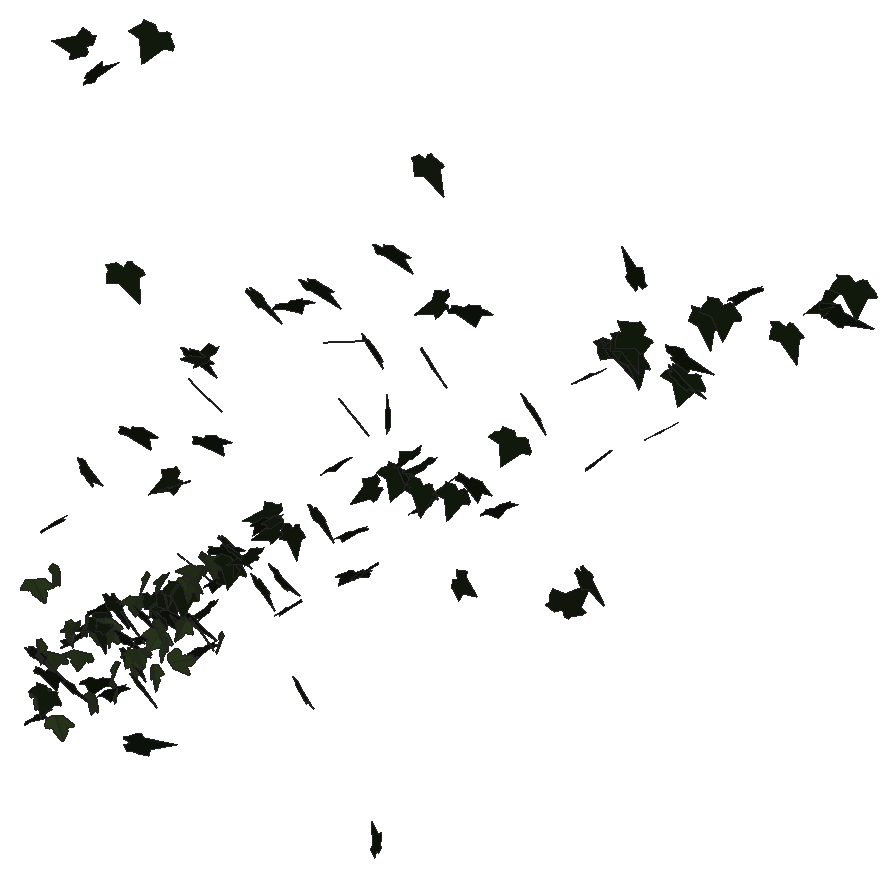
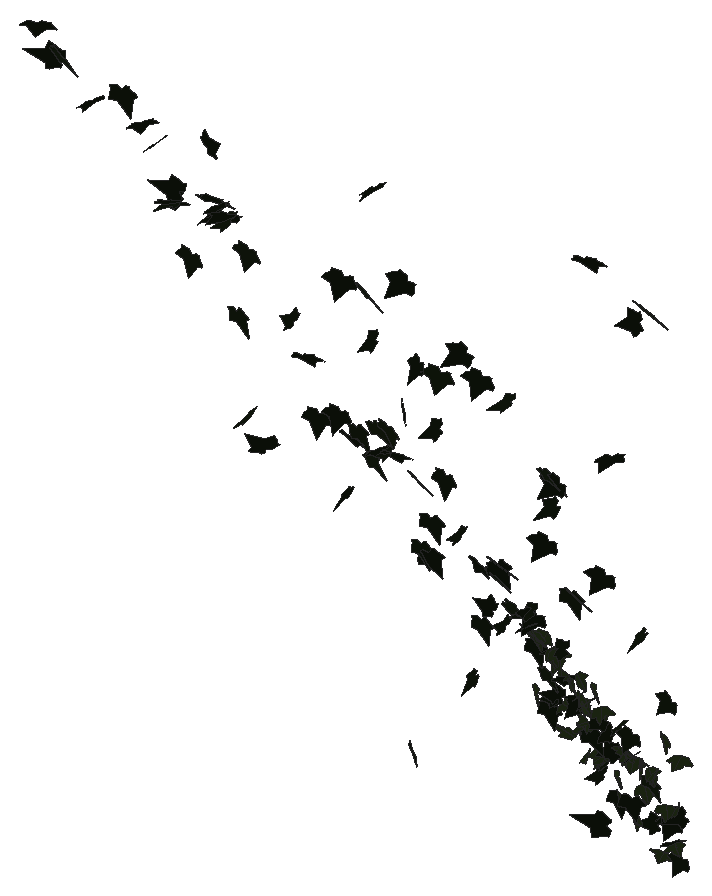
# SketchUp Ruby script. Lengths in inches.
U = 1.inch
M = Sketchup.active_model
def pt(a) = Geom::Point3d.new(a.map { |v| v * U })
def face(e, loops, mat)
  f = e.add_face(loops[0].map { |a| pt(a) })
  loops[1..].each { |l| e.add_face(l.map { |a| pt(a) }).erase! }
  f.material = f.back_material = mat if mat
  f
end
# faces: each face lists its corners as indices into pts; further lists are holes
def faces(e, pts, list, mat = nil) = list.each { |f| face(e, (f[0].is_a?(Array) ? f : [f]).map { |l| l.map { |i| pts[i] } }, mat) }
# xy, xz, yz: faces in a plane at the given z, y or x. An outline is a flat list of corners, or four numbers for a rectangle; further outlines are holes
def ring(l) = l.size == 4 ? [[l[0], l[1]], [l[2], l[1]], [l[2], l[3]], [l[0], l[3]]] : l.each_slice(2).to_a
def flat(e, list, mat, &to3) = list.each { |f| face(e, (f[0].is_a?(Array) ? f : [f]).map { |l| ring(l).map { |u, v| to3.(u, v) } }, mat) }
def xy(e, z, list, mat = nil) = flat(e, list, mat) { |x, y| [x, y, z] }
def xz(e, y, list, mat = nil) = flat(e, list, mat) { |x, z| [x, y, z] }
def yz(e, x, list, mat = nil) = flat(e, list, mat) { |y, z| [x, y, z] }
def lines(e, pts, list) = list.each { |a, b| e.add_line(pt(pts[a]), pt(pts[b])) }
# prism: a flat outline (further loops are holes) pulled along v
def prism(e, loops, v, mat = nil)
  f = face(e, loops, mat); d = Geom::Vector3d.new(v.map { |x| x * U })
  f.pushpull(f.normal.samedirection?(d) ? d.length : -d.length)
end
def box(e, o, s, mat = nil) = prism(e, [[o, [o[0] + s[0], o[1], o[2]], [o[0] + s[0], o[1] + s[1], o[2]], [o[0], o[1] + s[1], o[2]]]], [0, 0, s[2]], mat)
def at(x, y, z, deg = 0) = Geom::Transformation.translation(pt([x, y, z])) * Geom::Transformation.rotation(ORIGIN, Z_AXIS, deg.degrees)
def axes(o, x, y, z) = Geom::Transformation.new([*x, 0, *y, 0, *z, 0, *pt(o).to_a, 1])
def part(name) = M.definitions.add(name)
# library, detail: a bought-in or finely detailed component or shape, given as its bounding box
def library(name, o, s) = part(name).tap { |d| box(d.entities, o, s) }
def detail(e, o, s) = box(e.add_group.entities, o, s)
def put(e, d, t, mat = nil) = e.add_instance(d, t).tap { |i| i.material = mat if mat }
def group(e, t, mat = nil) = e.add_group.tap { |g| g.transformation = t; g.material = mat if mat }.entities
root = M.entities
M.materials.add("1026 AP 7946 SUNNY SIDE UP").color = [254, 231, 186]
M.materials.add("efeu1").color = [18, 25, 13]
M.materials.add("efeu2").color = [43, 57, 29]
c1 = part("ivyleaf_10")
p = [[0,0.5,-0.03],[-0.0625,2.02,-0.43],[-0.19,2.01,-0.46],[-0.54,1.05,-0.29],[-0.52,0.625,-0.18],[-0.83,0.76,-0.28],
  [-1.16,0.64,-0.33],[-1.15,0.33,-0.24],[-0.77,-0.39,0.02],[-0.3,-0.51,0.16],[0.04,-0.48,0.23],[-0.02,2.01,-0.4375],
  [-0.06,2.01,-0.43],[0.04,-0.49,0.23],[0.67,-0.49,0.14],[1.38,0.36,-0.2],[1.375,0.51,-0.24],[0.81,0.65,-0.19],
  [0.62,0.59,-0.15],[0.6,1.09,-0.28],[0.5,1.23,-0.31]]
faces(c1.entities,p,[[0,1,2,3,4,5,6,7,8,9,10],[11,12,0,13,14,15,16,17,18,19,20]],"efeu2")
c2 = part("ivyleaf_9")
p = [[1.54,2.16,1.25],[1.36,2.04,1.19],[-0.21,0.99,0.68],[-0.71,1.11,0.82],[-0.85,0.86,0.67],[-0.8,0.17,0.21],
  [-0.9,-0.01,0.1],[-0.67,-0.16,-0.02],[-0.08,-0.08,-0.05],[-0.03,-0.6,-0.4],[0.65,-0.88,-0.66],[0.83,-0.6,-0.49],
  [1.29,-0.42,-0.43],[1.8125,-0.07,-0.26],[1.21,0.44,0.15]]
faces(c2.entities,p,[[0,1,2,3,4,5,6,7,8,9,10,11,12,13,14]],"efeu1")
put(root,c1,axes([152.7,212.68,300.75],[-0.46729,-0.23939,-0.10574],[0.24139,-0.0375,-0.37295],[0.32982,-0.31172,0.12315]),"1026 AP 7946 SUNNY SIDE UP")
put(root,c2,axes([152.8,212.41,294.52],[0.19714,0.31739,0.16916],[0.09359,0.15111,-0.35068],[-0.55274,0.13879,0.00096]),"1026 AP 7946 SUNNY SIDE UP")
put(root,c1,axes([152.82,212.89,295.55],[0.30918,0.29061,-0.12024],[-0.13325,-0.08531,-0.36131],[-0.47507,0.21306,0.02309]),"1026 AP 7946 SUNNY SIDE UP")
put(root,c2,axes([152.45,212.77,297.4],[0.57206,-0.07756,0.06933],[0.08895,-0.05728,-0.38092],[0.13529,0.3656,-0.04269]),"1026 AP 7946 SUNNY SIDE UP")
put(root,c1,axes([152.77,212.8,297.81],[-0.08655,0.35409,-0.1255],[0.01107,-0.12416,-0.3697],[-0.58974,-0.05429,0.01148]),"1026 AP 7946 SUNNY SIDE UP")
put(root,c2,axes([153.16,212.88,295.63],[-0.25478,-0.32974,0.04474],[0.01184,-0.05401,-0.37752],[0.52322,-0.15934,0.03033]),"1026 AP 7946 SUNNY SIDE UP")
put(root,c2,axes([153.25,212.65,296.75],[0.51975,0.11539,-0.12956],[-0.17017,-0.07208,-0.35973],[-0.2085,0.34647,-0.02935]),"1026 AP 7946 SUNNY SIDE UP")
put(root,c1,axes([153.52,212.82,297.53],[-0.51807,-0.17242,0.03289],[-0.02153,-0.04451,-0.38185],[0.27517,-0.32811,0.03204]),"1026 AP 7946 SUNNY SIDE UP")
put(root,c2,axes([153.55,212.47,303.86],[0.22967,0.2776,0.26829],[0.13322,0.24652,-0.32016],[-0.58177,0.16604,0.0326]),"1026 AP 7946 SUNNY SIDE UP")
put(root,c1,axes([153.77,212.6875,301.67],[0.42896,-0.28302,-0.06521],[0.00837,0.08964,-0.39882],[0.4554,0.26494,0.06876]),"1026 AP 7946 SUNNY SIDE UP")
put(root,c1,axes([153.8,212.67,294.61],[0.5271,0.1067,0.13398],[0.20634,0.01343,-0.36139],[-0.16433,0.35909,-0.02401]),"1026 AP 7946 SUNNY SIDE UP")
put(root,c2,axes([154.73,212.72,298.75],[-0.13124,0.37251,0.05344],[-0.11374,0.03409,-0.38775],[-0.57989,-0.09099,0.06396]),"1026 AP 7946 SUNNY SIDE UP")
put(root,c1,axes([154.41,212.6875,299.27],[-0.05091,0.38742,-0.02757],[-0.00042,-0.02908,-0.40067],[-0.61088,-0.03226,0.00257]),"1026 AP 7946 SUNNY SIDE UP")
put(root,c1,axes([154.61,212.78,299.37],[-0.08768,-0.38044,0.04128],[-0.0053,-0.04219,-0.39635],[0.60185,-0.0558,0.00253]),"1026 AP 7946 SUNNY SIDE UP")
put(root,c2,axes([154.125,212.89,296.4],[0.43646,-0.17986,0.1778],[0.2205,-0.10272,-0.34122],[0.32539,0.31086,-0.00725]),"1026 AP 7946 SUNNY SIDE UP")
put(root,c2,axes([155.28,212.65,327.21],[-0.43062,0.331,0.19807],[-0.30187,0.08317,-0.43297],[-0.51901,-0.323,0.08749]),"1026 AP 7946 SUNNY SIDE UP")
put(root,c1,axes([155.05,212.71,298.16],[-0.45669,-0.23847,0.06481],[-0.04426,-0.06659,-0.38603],[0.38582,-0.28992,0.03243]),"1026 AP 7946 SUNNY SIDE UP")
put(root,c1,axes([155.23,212.79,299.65],[0.16583,-0.3476,-0.13742],[0.0593,0.14591,-0.36556],[0.5813,0.08427,0.07649]),"1026 AP 7946 SUNNY SIDE UP")
put(root,c2,axes([155.34,212.46,307.31],[0.47061,-0.11988,-0.26885],[-0.29648,0.20104,-0.31756],[0.33932,0.34192,0.0954]),"1026 AP 7946 SUNNY SIDE UP")
put(root,c1,axes([155.68,212.71,296.28],[0.45432,-0.24443,-0.03533],[0.03609,0.07711,-0.38202],[0.38612,0.28039,0.07728]),"1026 AP 7946 SUNNY SIDE UP")
put(root,c2,axes([155.87,212.76,297.23],[0.21645,0.30392,-0.18263],[-0.09119,-0.17003,-0.34435],[-0.54706,0.14859,-0.01486]),"1026 AP 7946 SUNNY SIDE UP")
put(root,c1,axes([155.89,212.75,299.67],[-0.56757,-0.12501,-0.00205],[0.01887,-0.03075,-0.39224],[0.19567,-0.35965,0.03187]),"1026 AP 7946 SUNNY SIDE UP")
put(root,c2,axes([156.25,212.89,300.09],[-0.57953,0.1147,0.01403],[-0.0702,-0.10162,-0.38169],[-0.16737,-0.35452,0.11149]),"1026 AP 7946 SUNNY SIDE UP")
put(root,c2,axes([155.74,212.46,326.01],[0.20754,0.14293,0.43993],[0.40404,0.34051,-0.19762],[-0.58002,0.28834,0.01976]),"1026 AP 7946 SUNNY SIDE UP")
put(root,c2,axes([155.84,212.85,299.84],[0.07382,-0.38326,0.00387],[-0.01214,-0.00692,-0.39773],[0.60259,0.04681,-0.00849]),"1026 AP 7946 SUNNY SIDE UP")
put(root,c2,axes([156.17,212.43,300.89],[0.24256,0.34415,0.13491],[0.07431,0.12017,-0.38778],[-0.57311,0.16123,0.00682]),"1026 AP 7946 SUNNY SIDE UP")
put(root,c1,axes([156.32,212.91,299.84],[-0.38888,0.27151,-0.11323],[-0.00772,-0.14955,-0.36498],[-0.46143,-0.22632,0.10153]),"1026 AP 7946 SUNNY SIDE UP")
put(root,c1,axes([156.26,212.87,300.02],[-0.51042,-0.01549,-0.21285],[0.30783,-0.14824,-0.30641],[-0.10626,-0.35504,0.13477]),"1026 AP 7946 SUNNY SIDE UP")
put(root,c2,axes([156.75,212.6875,297.1],[0.13138,0.36736,-0.06784],[-0.00435,-0.06901,-0.38831],[-0.58742,0.08267,-0.0123]),"1026 AP 7946 SUNNY SIDE UP")
put(root,c1,axes([156.85,212.71,297.16],[0.31676,-0.29345,-0.14725],[-0.00811,0.16321,-0.35589],[0.51203,0.18412,0.08545]),"1026 AP 7946 SUNNY SIDE UP")
put(root,c1,axes([156.875,212.77,298.21],[0.29073,-0.29999,0.15478],[0.10385,-0.13763,-0.36352],[0.51846,0.19579,-0.01398]),"1026 AP 7946 SUNNY SIDE UP")
put(root,c2,axes([156.65,212.76,301.36],[0.26644,-0.35465,-0.03665],[0.00569,0.03888,-0.40417],[0.56012,0.16831,0.02154]),"1026 AP 7946 SUNNY SIDE UP")
put(root,c2,axes([156.99,212.8,299.73],[0.53572,-0.10857,0.15097],[0.21563,-0.05418,-0.36857],[0.19023,0.36715,-0.00737]),"1026 AP 7946 SUNNY SIDE UP")
put(root,c2,axes([157.38,212.64,317.38],[-0.05948,-0.3931,-0.27522],[0.04293,0.26351,-0.4053],[0.74414,-0.04663,0.00138]),"1026 AP 7946 SUNNY SIDE UP")
put(root,c2,axes([157.42,212.68,300.78],[0.52894,-0.17181,-0.08172],[-0.13092,0.00871,-0.38789],[0.26649,0.34528,-0.02836]),"1026 AP 7946 SUNNY SIDE UP")
put(root,c2,axes([157.41,212.89,299.02],[0.2769,-0.33735,-0.04186],[-0.00069,0.04339,-0.39126],[0.53393,0.175,0.0212]),"1026 AP 7946 SUNNY SIDE UP")
put(root,c1,axes([157.8,212.68,298.99],[0.1388,0.37292,0.00465],[0.00614,0.00153,-0.39477],[-0.58635,0.08829,-0.00304]),"1026 AP 7946 SUNNY SIDE UP")
put(root,c1,axes([158,212.72,301.83],[-0.36108,-0.32324,0.00717],[0.0594,-0.03753,-0.4051],[0.50497,-0.22672,0.05278]),"1026 AP 7946 SUNNY SIDE UP")
put(root,c1,axes([157.95,212.79,299.27],[-0.4155,-0.2615,-0.10896],[0.16797,0.03919,-0.37988],[0.40957,-0.28136,0.04525]),"1026 AP 7946 SUNNY SIDE UP")
put(root,c2,axes([157.94,212.5,309.96],[0.59891,0.18821,-0.04457],[-0.03454,-0.05519,-0.4361],[-0.30207,0.37947,-0.0385]),"1026 AP 7946 SUNNY SIDE UP")
put(root,c2,axes([157.87,212.73,301.35],[0.58966,-0.11928,0.0099],[0.00204,-0.02978,-0.40455],[0.18824,0.37396,-0.02663]),"1026 AP 7946 SUNNY SIDE UP")
put(root,c2,axes([157.95,212.72,298],[0.4141,-0.27586,0.05587],[0.04931,-0.04719,-0.39305],[0.43979,0.26504,-0.00854]),"1026 AP 7946 SUNNY SIDE UP")
put(root,c2,axes([157.81,212.67,294.98],[0.3582,0.23468,-0.33496],[0.26032,0.2872,0.33337],[0.57614,-0.27568,0.05762]),"1026 AP 7946 SUNNY SIDE UP")
put(root,c2,axes([158.58,212.78,300.3],[0.00189,0.34594,-0.17418],[-0.09662,-0.16868,-0.35292],[-0.59907,0.0283,0.05637]),"1026 AP 7946 SUNNY SIDE UP")
put(root,c1,axes([158.51,212.73,302.99],[0.27732,-0.35602,0.04732],[0.01368,-0.04918,-0.40934],[0.56469,0.17603,-0.01333]),"1026 AP 7946 SUNNY SIDE UP")
put(root,c2,axes([158.91,212.93,328.98],[-0.61459,-0.23999,-0.10214],[0.16248,0.01794,-0.47078],[0.37369,-0.4025,0.03672]),"1026 AP 7946 SUNNY SIDE UP")
put(root,c1,axes([158.97,212.92,301.96],[0.11767,-0.35972,0.13554],[0.00968,-0.13498,-0.37874],[0.6033,0.07233,-0.02036]),"1026 AP 7946 SUNNY SIDE UP")
put(root,c1,axes([159.04,212.84,300.49],[0.42453,0.21919,-0.17855],[-0.17801,-0.13641,-0.35764],[-0.40303,0.29113,-0.03011]),"1026 AP 7946 SUNNY SIDE UP")
put(root,c2,axes([158.79,212.79,302.14],[0.15813,-0.37337,-0.08929],[-0.00698,0.08627,-0.39743],[0.60191,0.09909,0.01885]),"1026 AP 7946 SUNNY SIDE UP")
put(root,c1,axes([158.99,212.67,298.83],[-0.01287,0.36928,-0.12262],[0.01072,-0.12099,-0.38121],[-0.611,-0.0099,-0.0041]),"1026 AP 7946 SUNNY SIDE UP")
put(root,c1,axes([158.96,212.875,300.89],[-0.33648,0.16972,-0.28139],[0.25159,-0.22971,-0.27656],[-0.4401,-0.26108,0.05704]),"1026 AP 7946 SUNNY SIDE UP")
put(root,c1,axes([159.42,212.76,303.37],[0.04162,-0.38816,0.09481],[-0.00016,-0.09445,-0.40131],[0.62808,0.0257,-0.00639]),"1026 AP 7946 SUNNY SIDE UP")
put(root,c1,axes([159.26,212.85,302.29],[0.45646,-0.25907,0.01379],[0.12077,0.06448,-0.38721],[0.38974,0.28343,0.10383]),"1026 AP 7946 SUNNY SIDE UP")
put(root,c1,axes([159.41,212.78,300.25],[0.41338,-0.25873,0.13047],[0.14465,-0.08917,-0.38051],[0.43031,0.27853,0.00257]),"1026 AP 7946 SUNNY SIDE UP")
put(root,c2,axes([159.375,212.9375,302.33],[0.17142,-0.3735,-0.04847],[-0.00315,0.0462,-0.4004],[0.59151,0.10848,0.01191]),"1026 AP 7946 SUNNY SIDE UP")
put(root,c2,axes([159.45,212.55,301.73],[0.5745,0.13316,0.00691],[0.02877,-0.03289,-0.39897],[-0.20761,0.36393,-0.03615]),"1026 AP 7946 SUNNY SIDE UP")
put(root,c2,axes([160.05,212.71,308.28],[-0.60582,0.15009,-0.05909],[0.05843,-0.06399,-0.42374],[-0.2463,-0.38436,0.04482]),"1026 AP 7946 SUNNY SIDE UP")
put(root,c2,axes([160.15,212.58,308.07],[-0.00918,0.41343,-0.0504],[-0.1097,-0.05152,-0.42012],[-0.64581,0.00287,0.07208]),"1026 AP 7946 SUNNY SIDE UP")
put(root,c1,axes([159.97,212.875,303.03],[0.20624,-0.35931,0.09999],[0.04618,-0.09476,-0.39458],[0.58426,0.13433,-0.00411]),"1026 AP 7946 SUNNY SIDE UP")
put(root,c1,axes([160.41,212.88,301.46],[0.12824,0.268,-0.27827],[-0.12859,-0.25904,-0.2901],[-0.58607,0.11548,0.00276]),"1026 AP 7946 SUNNY SIDE UP")
put(root,c2,axes([160.34,212.84,303.1],[-0.26243,-0.35073,-0.08435],[0.08768,0.06178,-0.39906],[0.55878,-0.17442,0.023]),"1026 AP 7946 SUNNY SIDE UP")
put(root,c1,axes([160.11,212.68,299.65],[0.34344,-0.0708,-0.32735],[0.5086,0.00823,0.22749],[-0.05226,-0.38517,0.0627]),"1026 AP 7946 SUNNY SIDE UP")
put(root,c1,axes([160.46,212.88,303.42],[0.53169,-0.14793,0.14952],[0.22029,-0.04367,-0.38017],[0.24138,0.3657,0.01761]),"1026 AP 7946 SUNNY SIDE UP")
put(root,c1,axes([160.96,212.76,304.3],[-0.33182,-0.33884,0.04538],[-0.01755,-0.04717,-0.41121],[0.53739,-0.21076,0.01459]),"1026 AP 7946 SUNNY SIDE UP")
put(root,c2,axes([160.49,212.72,304.66],[0.53187,-0.21142,0.07686],[0.14165,0.00216,-0.40785],[0.32351,0.34664,0.05221]),"1026 AP 7946 SUNNY SIDE UP")
put(root,c1,axes([161.04,212.72,303.77],[-0.46215,0.26408,0.00666],[-0.03425,-0.01682,-0.4062],[-0.4139,-0.29347,0.02617]),"1026 AP 7946 SUNNY SIDE UP")
put(root,c2,axes([160.66,212.89,301.81],[0.4038,-0.19764,0.22517],[0.25112,-0.15208,-0.33414],[0.39096,0.30181,-0.01795]),"1026 AP 7946 SUNNY SIDE UP")
put(root,c1,axes([161.25,212.85,304.29],[-0.15116,-0.38339,0.06252],[-0.00319,-0.06426,-0.40733],[0.61088,-0.0952,0.01334]),"1026 AP 7946 SUNNY SIDE UP")
put(root,c2,axes([160.93,212.73,314.58],[0.67807,0.01024,-0.03177],[-0.04706,-0.03674,-0.44305],[-0.02013,0.43078,-0.03449]),"1026 AP 7946 SUNNY SIDE UP")
put(root,c2,axes([160.91,212.86,301.7],[0.40348,-0.27515,0.11033],[0.0736,-0.10427,-0.38648],[0.45931,0.25841,-0.03499]),"1026 AP 7946 SUNNY SIDE UP")
put(root,c2,axes([161.53,212.66,300.8],[0.04597,0.38632,-0.08013],[-0.00356,-0.08003,-0.39958],[-0.62033,0.02909,-0.00364]),"1026 AP 7946 SUNNY SIDE UP")
put(root,c2,axes([161.88,212.55,314.83],[-0.37367,0.36503,0.04298],[-0.15058,-0.01602,-0.43943],[-0.55737,-0.24039,0.0899]),"1026 AP 7946 SUNNY SIDE UP")
put(root,c2,axes([161.18,212.67,313.1],[0.61997,-0.14891,-0.09355],[-0.10888,0.07012,-0.4318],[0.25095,0.39829,0.04377]),"1026 AP 7946 SUNNY SIDE UP")
put(root,c2,axes([161.9375,212.59,302.82],[-0.3217,0.33521,-0.05269],[0.01851,-0.0549,-0.40445],[-0.53332,-0.2041,0.01775]),"1026 AP 7946 SUNNY SIDE UP")
put(root,c1,axes([161.82,212.73,305.09],[-0.58071,0.15328,-0.05551],[0.05478,-0.05817,-0.4102],[-0.25,-0.36879,0.03905]),"1026 AP 7946 SUNNY SIDE UP")
put(root,c2,axes([161.68,212.6875,310.77],[0.53747,0.24858,-0.00239],[0.02249,-0.02599,-0.4345],[-0.39027,0.34084,-0.02833]),"1026 AP 7946 SUNNY SIDE UP")
put(root,c2,axes([162.4,212.7,304.34],[0.03325,0.38542,-0.09628],[0.01526,-0.09625,-0.39793],[-0.62423,0.01817,-0.01486]),"1026 AP 7946 SUNNY SIDE UP")
put(root,c1,axes([162.41,212.82,304.99],[0.5351,-0.1611,-0.15065],[-0.17211,0.10592,-0.3844],[0.29455,0.35455,0.04907]),"1026 AP 7946 SUNNY SIDE UP")
put(root,c1,axes([162.51,212.67,301.55],[0.21381,-0.36771,-0.07313],[-0.01896,0.06897,-0.40328],[0.58794,0.13594,0.01359]),"1026 AP 7946 SUNNY SIDE UP")
put(root,c2,axes([163.03,212.59,304.78],[-0.21944,0.22615,0.30875],[-0.30986,0.22643,-0.27039],[-0.50061,-0.23928,0.03203]),"1026 AP 7946 SUNNY SIDE UP")
put(root,c2,axes([162.5625,212.58,305.93],[0.47466,0.27496,0.00617],[0.03246,-0.0161,-0.41991],[-0.43119,0.30147,-0.02482]),"1026 AP 7946 SUNNY SIDE UP")
put(root,c2,axes([162.91,212.91,305.24],[-0.17859,-0.3775,0.07414],[0.00444,-0.07809,-0.40578],[0.6049,-0.11088,0.02487]),"1026 AP 7946 SUNNY SIDE UP")
put(root,c2,axes([162.66,212.75,306.23],[0.46748,-0.28204,0.01077],[0.06641,0.02713,-0.41902],[0.4389,0.29631,0.05193]),"1026 AP 7946 SUNNY SIDE UP")
put(root,c2,axes([164.27,212.75,306.1],[-0.44911,0.27404,-0.07304],[-0.05942,-0.13876,-0.38798],[-0.44172,-0.25995,0.12646]),"1026 AP 7946 SUNNY SIDE UP")
put(root,c2,axes([164.12,212.84,318.45],[0.49112,-0.31156,-0.04615],[0.0337,0.08159,-0.44782],[0.4934,0.30455,0.07653]),"1026 AP 7946 SUNNY SIDE UP")
put(root,c2,axes([164.38,212.88,304.82],[0.26919,-0.34088,0.12582],[0.06982,-0.11647,-0.39346],[0.56612,0.17646,-0.0113]),"1026 AP 7946 SUNNY SIDE UP")
put(root,c2,axes([165.05,212.62,308.16],[-0.01598,0.36242,-0.21471],[-0.00954,-0.21065,-0.37459],[-0.65894,-0.00574,0.01063]),"1026 AP 7946 SUNNY SIDE UP")
put(root,c2,axes([165.34,212.74,308.41],[-0.55605,0.20572,0.06575],[-0.14153,-0.03208,-0.41505],[-0.30709,-0.3577,0.07224]),"1026 AP 7946 SUNNY SIDE UP")
put(root,c2,axes([165.45,212.76,307.72],[-0.49245,0.25893,-0.00537],[-0.02396,-0.02888,-0.41751],[-0.40658,-0.31192,0.03111]),"1026 AP 7946 SUNNY SIDE UP")
put(root,c2,axes([165.33,212.85,305.48],[0.27201,-0.19807,0.31435],[0.27135,-0.25417,-0.27125],[0.50524,0.24314,-0.02355]),"1026 AP 7946 SUNNY SIDE UP")
put(root,c2,axes([166.15,212.64,304.38],[-0.05855,0.40378,-0.03858],[-0.00009,-0.03991,-0.41796],[-0.63798,-0.03705,0.0036]),"1026 AP 7946 SUNNY SIDE UP")
put(root,c2,axes([166.32,212.41,318.96],[0.39403,0.38151,0.03962],[0.00993,0.03924,-0.46971],[-0.60252,0.25014,0.01817]),"1026 AP 7946 SUNNY SIDE UP")
put(root,c2,axes([166.14,212.89,307.9375],[-0.33924,-0.06258,-0.35349],[0.54663,-0.01143,-0.22334],[0.037,-0.40486,0.05852]),"1026 AP 7946 SUNNY SIDE UP")
put(root,c2,axes([166.65,212.59,300.84],[0.48463,-0.16227,-0.23128],[-0.30269,0.11412,-0.35803],[0.31157,0.36326,0.01193]),"1026 AP 7946 SUNNY SIDE UP")
put(root,c2,axes([167.32,212.6,320.17],[0.7052,0.033,0.04025],[0.0654,-0.03749,-0.46163],[-0.04642,0.44861,-0.03889]),"1026 AP 7946 SUNNY SIDE UP")
put(root,c2,axes([167.39,212.85,309.24],[0.33162,-0.356,0.04455],[0.01721,-0.0461,-0.42631],[0.56403,0.21072,-0.01319]),"1026 AP 7946 SUNNY SIDE UP")
put(root,c2,axes([168.77,212.4,312.11],[0.08083,0.42761,0.08282],[0.02463,0.07663,-0.4432],[-0.68302,0.05337,-0.00618]),"1026 AP 7946 SUNNY SIDE UP")
put(root,c2,axes([169.15,212.32,318.2],[0.38088,0.3757,0.04108],[-0.17009,0.11201,-0.43276],[-0.56884,0.21807,0.15691]),"1026 AP 7946 SUNNY SIDE UP")
put(root,c2,axes([169.66,212.66,307.23],[0.01815,0.35709,-0.21926],[-0.11508,-0.20987,-0.3646],[-0.64512,0.04748,0.05887]),"1026 AP 7946 SUNNY SIDE UP")
put(root,c2,axes([169.65,212.48,309.24],[0.02787,0.40748,-0.08387],[-0.07641,-0.0812,-0.41819],[-0.64963,0.02703,0.04559]),"1026 AP 7946 SUNNY SIDE UP")
put(root,c2,axes([169.06,212.65,315],[0.5555,-0.25872,0.01002],[-0.01249,-0.02976,-0.45031],[0.407,0.3522,-0.0275]),"1026 AP 7946 SUNNY SIDE UP")
put(root,c2,axes([170.21,212.62,307.55],[-0.0683,0.41323,-0.04306],[0.00011,-0.04437,-0.42828],[-0.65346,-0.0432,0.00443]),"1026 AP 7946 SUNNY SIDE UP")
put(root,c2,axes([170.64,212.76,311.62],[-0.59152,0.15712,-0.09548],[0.10786,-0.07718,-0.41803],[-0.26656,-0.37989,0.04274]),"1026 AP 7946 SUNNY SIDE UP")
put(root,c2,axes([170.43,212.59,318.45],[0.58026,-0.13276,-0.22041],[-0.33683,0.03143,-0.40196],[0.20615,0.42502,-0.03638]),"1026 AP 7946 SUNNY SIDE UP")
put(root,c2,axes([170.9,212.49,294.61],[-0.01747,0.0683,0.43341],[-0.05978,0.41862,-0.06866],[-0.66691,-0.03931,-0.0052]),"1026 AP 7946 SUNNY SIDE UP")
put(root,c2,axes([171.51,212.49,314.97],[-0.00594,-0.01905,0.45631],[0.02532,0.44276,0.02235],[-0.69683,0.01625,-0.00308]),"1026 AP 7946 SUNNY SIDE UP")
put(root,c2,axes([171.25,212.67,323.17],[0.70937,0.08541,-0.00261],[0.00798,-0.04296,-0.47117],[-0.13415,0.4491,-0.04183]),"1026 AP 7946 SUNNY SIDE UP")
put(root,c2,axes([171.91,212.91,312.64],[-0.52255,-0.24363,-0.10306],[0.19955,-0.00945,-0.41641],[0.36195,-0.34653,0.08078]),"1026 AP 7946 SUNNY SIDE UP")
put(root,c2,axes([172.61,212.46,313.74],[-0.03574,0.38544,0.20355],[-0.12697,0.18843,-0.3915],[-0.66753,-0.05648,0.06357]),"1026 AP 7946 SUNNY SIDE UP")
put(root,c2,axes([172.15,212.86,312.67],[0.36339,-0.35578,0.02761],[-0.00777,-0.03752,-0.43655],[0.5612,0.22985,-0.02392]),"1026 AP 7946 SUNNY SIDE UP")
put(root,c2,axes([173.42,212.58,313.67],[-0.30869,0.37426,-0.04619],[-0.09475,-0.08338,-0.42553],[-0.58548,-0.18383,0.09322]),"1026 AP 7946 SUNNY SIDE UP")
put(root,c2,axes([173.04,212.89,312.42],[-0.15493,-0.41201,0.01733],[-0.00821,-0.01846,-0.43652],[0.64849,-0.09866,-0.00139]),"1026 AP 7946 SUNNY SIDE UP")
put(root,c2,axes([173.5,212.83,311.84],[-0.35511,0.34873,-0.08283],[0.02515,-0.08748,-0.42714],[-0.56288,-0.22392,0.03317]),"1026 AP 7946 SUNNY SIDE UP")
put(root,c2,axes([173.39,212.67,328.09],[0.12999,-0.42919,-0.19171],[-0.02438,0.18389,-0.44881],[0.73364,0.08215,0.01906]),"1026 AP 7946 SUNNY SIDE UP")
put(root,c2,axes([173.37,212.65,318.89],[0.53439,-0.29377,-0.05444],[-0.11175,-0.00444,-0.46],[0.45537,0.34366,-0.049]),"1026 AP 7946 SUNNY SIDE UP")
put(root,c2,axes([174.3,212.65,321.7],[-0.56995,0.27653,-0.02144],[0.00703,-0.031,-0.46932],[-0.43619,-0.36184,0.02045]),"1026 AP 7946 SUNNY SIDE UP")
put(root,c2,axes([174.47,212.6875,313.12],[-0.19511,0.40179,-0.06997],[0.00539,-0.07235,-0.43325],[-0.64133,-0.12285,0.01765]),"1026 AP 7946 SUNNY SIDE UP")
put(root,c2,axes([174.76,213,312.72],[-0.54818,-0.10662,-0.22817],[0.37105,-0.04118,-0.36347],[0.10512,-0.41065,0.0931]),"1026 AP 7946 SUNNY SIDE UP")
put(root,c2,axes([175.3,212.42,308.97],[0.25398,-0.14692,-0.3796],[-0.30847,0.31518,-0.21671],[0.54073,0.24881,0.05467]),"1026 AP 7946 SUNNY SIDE UP")
put(root,c2,axes([175.55,212.59,321.89],[0.51419,0.30677,-0.09553],[-0.08492,-0.08035,-0.46187],[-0.49752,0.33076,-0.01989]),"1026 AP 7946 SUNNY SIDE UP")
put(root,c2,axes([175.67,212.72,313.7],[0.59042,0.07976,-0.19661],[-0.27576,-0.08869,-0.39324],[-0.17368,0.41197,-0.04399]),"1026 AP 7946 SUNNY SIDE UP")
put(root,c2,axes([177.19,212.59,312.98],[0.20598,0.41455,-0.00301],[0.00855,-0.00725,-0.44786],[-0.65184,0.1309,-0.00682]),"1026 AP 7946 SUNNY SIDE UP")
put(root,c2,axes([177.97,212.87,316.41],[-0.55351,-0.24889,-0.06782],[0.12424,-0.0008,-0.44163],[0.38468,-0.35786,0.04505]),"1026 AP 7946 SUNNY SIDE UP")
put(root,c2,axes([178.71,212.9,318.25],[0.26591,-0.33921,0.22985],[0.12142,-0.21254,-0.39105],[0.62847,0.18458,-0.0217]),"1026 AP 7946 SUNNY SIDE UP")
put(root,c2,axes([180.93,212.4,309.59],[-0.27003,-0.00987,0.46408],[0.65697,0.17717,0.1691],[-0.26551,0.44842,-0.05356]),"1026 AP 7946 SUNNY SIDE UP")
put(root,c2,axes([181.73,212.65,311.42],[0.39014,-0.3454,-0.15434],[-0.11908,0.12758,-0.4372],[0.57866,0.25913,0.0141]),"1026 AP 7946 SUNNY SIDE UP")
put(root,c2,axes([182.17,212.32,321.04],[0.18332,0.40025,0.16949],[-0.05703,0.17653,-0.42076],[-0.67669,0.09355,0.08137]),"1026 AP 7946 SUNNY SIDE UP")
put(root,c2,axes([182.71,212.56,317.23],[-0.19089,0.43042,-0.0221],[0.00081,-0.02468,-0.46081],[-0.67783,-0.12125,0.00567]),"1026 AP 7946 SUNNY SIDE UP")
put(root,c2,axes([183.1,212.73,322.72],[0.41623,-0.37401,-0.01348],[0.02471,0.02452,-0.47108],[0.58783,0.2638,0.02934]),"1026 AP 7946 SUNNY SIDE UP")
put(root,c2,axes([183.29,212.69,322.96],[0.00565,-0.31315,-0.34641],[0.26605,0.31175,-0.29699],[0.66953,-0.12124,0.12094]),"1026 AP 7946 SUNNY SIDE UP")
put(root,c2,axes([183.89,212.77,323.3125],[0.03906,-0.43058,-0.16314],[-0.01511,0.15562,-0.44341],[0.7199,0.02663,-0.00046]),"1026 AP 7946 SUNNY SIDE UP")
put(root,c2,axes([184.65,212.84,323.67],[-0.67277,-0.05063,0.14447],[-0.20126,-0.0955,-0.43748],[0.12107,-0.44011,0.07557]),"1026 AP 7946 SUNNY SIDE UP")
put(root,c2,axes([184.8,212.43,326.46],[0.06754,-0.06183,0.48469],[-0.26445,0.44014,0.07793],[-0.6983,-0.17266,0.01737]),"1026 AP 7946 SUNNY SIDE UP")
put(root,c2,axes([184.34,212.86,322.6],[-0.00245,-0.45299,0.03133],[-0.02587,-0.0329,-0.46656],[0.7137,-0.00275,-0.0168]),"1026 AP 7946 SUNNY SIDE UP")
put(root,c2,axes([185.82,212.5625,319.61],[0.14367,0.42006,0.15536],[-0.01005,0.15273,-0.44036],[-0.70045,0.08397,0.03818]),"1026 AP 7946 SUNNY SIDE UP")
put(root,c2,axes([186.72,212.53,322.74],[0.60415,-0.20845,-0.14169],[-0.08175,0.17802,-0.43026],[0.38303,0.36678,0.13165]),"1026 AP 7946 SUNNY SIDE UP")
put(root,c2,axes([187.06,212.93,322.58],[-0.47052,-0.33916,-0.05632],[0.13713,-0.00745,-0.46041],[0.522,-0.30376,0.07019]),"1026 AP 7946 SUNNY SIDE UP")
put(root,c2,axes([186.51,212.84,323.34],[0.40055,-0.1069,0.37281],[0.48417,-0.19475,-0.28323],[0.34454,0.39795,-0.03541]),"1026 AP 7946 SUNNY SIDE UP")
put(root,c2,axes([187.98,212.875,325.76],[0.04396,-0.45775,0.05477],[0.0002,-0.05586,-0.47276],[0.72508,0.02777,-0.00319]),"1026 AP 7946 SUNNY SIDE UP")
put(root,c2,axes([189.02,212.84,326.59],[-0.22937,-0.43739,-0.06312],[0.02582,0.05649,-0.47466],[0.69346,-0.14678,-0.00321]),"1026 AP 7946 SUNNY SIDE UP")
put(root,c2,axes([190.5,212.55,327.92],[0.0243,0.44894,-0.12342],[-0.03795,-0.12148,-0.46305],[-0.73067,0.02124,0.01995]),"1026 AP 7946 SUNNY SIDE UP")
put(root,c2,axes([192.38,212.8,326.75],[0.01849,-0.45434,-0.11277],[0.00991,0.10706,-0.4675],[0.73383,0.01,0.00916]),"1026 AP 7946 SUNNY SIDE UP")
put(root,c2,axes([194.82,212.75,328.91],[-0.52221,0.33217,-0.05117],[0.01522,-0.063,-0.48273],[-0.52834,-0.33013,0.03668]),"1026 AP 7946 SUNNY SIDE UP")
put(root,c2,axes([194.82,212.67,328.38],[0.43362,-0.05565,0.39454],[0.56903,-0.13065,-0.28854],[0.21703,0.45375,-0.03177]),"1026 AP 7946 SUNNY SIDE UP")
put(root,c2,axes([196.06,212.8,330.15],[-0.39275,-0.36179,-0.18887],[0.18361,0.13953,-0.45181],[0.60923,-0.27529,0.01441]),"1026 AP 7946 SUNNY SIDE UP")
